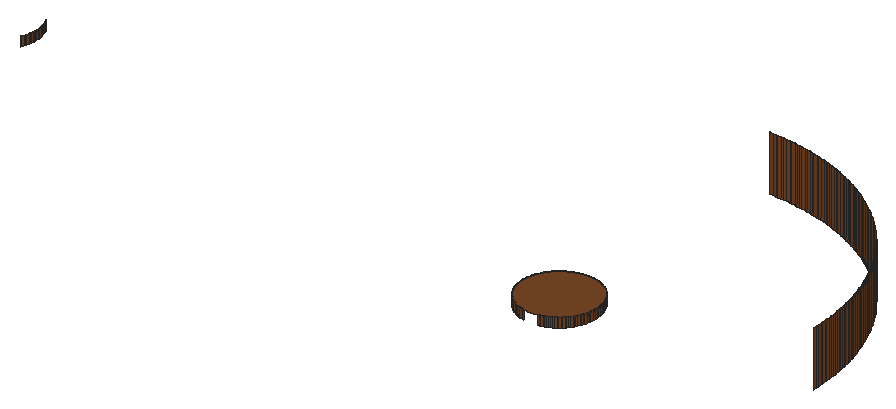
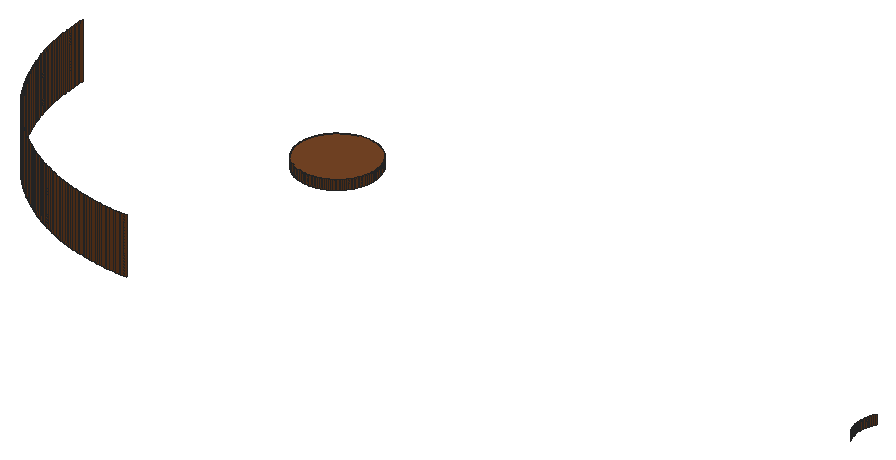
# SketchUp Ruby script. Lengths in inches.
U = 1.inch
M = Sketchup.active_model
def pt(a) = Geom::Point3d.new(a.map { |v| v * U })
def face(e, loops, mat)
  f = e.add_face(loops[0].map { |a| pt(a) })
  loops[1..].each { |l| e.add_face(l.map { |a| pt(a) }).erase! }
  f.material = f.back_material = mat if mat
  f
end
# faces: each face lists its corners as indices into pts; further lists are holes
def faces(e, pts, list, mat = nil) = list.each { |f| face(e, (f[0].is_a?(Array) ? f : [f]).map { |l| l.map { |i| pts[i] } }, mat) }
# xy, xz, yz: faces in a plane at the given z, y or x. An outline is a flat list of corners, or four numbers for a rectangle; further outlines are holes
def ring(l) = l.size == 4 ? [[l[0], l[1]], [l[2], l[1]], [l[2], l[3]], [l[0], l[3]]] : l.each_slice(2).to_a
def flat(e, list, mat, &to3) = list.each { |f| face(e, (f[0].is_a?(Array) ? f : [f]).map { |l| ring(l).map { |u, v| to3.(u, v) } }, mat) }
def xy(e, z, list, mat = nil) = flat(e, list, mat) { |x, y| [x, y, z] }
def xz(e, y, list, mat = nil) = flat(e, list, mat) { |x, z| [x, y, z] }
def yz(e, x, list, mat = nil) = flat(e, list, mat) { |y, z| [x, y, z] }
def lines(e, pts, list) = list.each { |a, b| e.add_line(pt(pts[a]), pt(pts[b])) }
# prism: a flat outline (further loops are holes) pulled along v
def prism(e, loops, v, mat = nil)
  f = face(e, loops, mat); d = Geom::Vector3d.new(v.map { |x| x * U })
  f.pushpull(f.normal.samedirection?(d) ? d.length : -d.length)
end
def box(e, o, s, mat = nil) = prism(e, [[o, [o[0] + s[0], o[1], o[2]], [o[0] + s[0], o[1] + s[1], o[2]], [o[0], o[1] + s[1], o[2]]]], [0, 0, s[2]], mat)
def at(x, y, z, deg = 0) = Geom::Transformation.translation(pt([x, y, z])) * Geom::Transformation.rotation(ORIGIN, Z_AXIS, deg.degrees)
def axes(o, x, y, z) = Geom::Transformation.new([*x, 0, *y, 0, *z, 0, *pt(o).to_a, 1])
def part(name) = M.definitions.add(name)
# library, detail: a bought-in or finely detailed component or shape, given as its bounding box
def library(name, o, s) = part(name).tap { |d| box(d.entities, o, s) }
def detail(e, o, s) = box(e.add_group.entities, o, s)
def put(e, d, t, mat = nil) = e.add_instance(d, t).tap { |i| i.material = mat if mat }
def group(e, t, mat = nil) = e.add_group.tap { |g| g.transformation = t; g.material = mat if mat }.entities
root = M.entities
M.materials.add("[Wood Veneer 01]3").color = [120, 70, 37]
xy(root,118.5,[[142.9,168,142.74,168.02,142.65,168.03,142.41,168.09,142.17,168.18,142.1,168.21,142.02,168.25,141.95,168.3,141.88,168.34,141.8125,168.39,141.75,168.44,141.68,168.5,141.62,168.55,141.5625,168.61,141.5,168.67,141.45,168.74,141.4,168.8,141.3,168.94,141.26,169.01,141.22,169.09,141.18,169.16,141.09,169.4,141.03,169.64,141.01,169.8,141,169.89,141,170.14,141.01,170.22,141.02,170.31,141.1,170.63,141.16,170.79,141.2,170.86,141.23,170.9375,141.27,171.01,141.47,171.29,141.52,171.35,141.64,171.47,141.7,171.52,141.77,171.58,141.84,171.625,141.9,171.67,141.98,171.72,142.05,171.76,142.125,171.8,142.2,171.83,142.44,171.92,142.6,171.96,142.68,171.97,142.76,171.99,142.85,171.99,142.93,172,143.1,172,143.26,171.98,143.35,171.97,143.59,171.91,143.83,171.82,143.9,171.79,143.98,171.75,144.05,171.7,144.12,171.66,144.1875,171.61,144.25,171.56,144.32,171.5,144.38,171.45,144.4375,171.39,144.5,171.33,144.55,171.26,144.6,171.2,144.7,171.06,144.74,170.99,144.78,170.91,144.82,170.84,144.91,170.6,144.97,170.36,144.99,170.2,145,170.11,145,169.86,144.99,169.78,144.98,169.69,144.9,169.37,144.84,169.21,144.8,169.14,144.77,169.0625,144.73,168.99,144.53,168.71,144.48,168.65,144.36,168.53,144.3,168.48,144.23,168.42,144.16,168.375,144.1,168.33,144.02,168.28,143.95,168.24,143.875,168.2,143.8,168.17,143.56,168.08,143.4,168.04,143.32,168.03,143.24,168.01,143.15,168.01,143.07,168]],"[Wood Veneer 01]3")
xz(root,171.99,[[142.76,118,142.85,118.5]],"[Wood Veneer 01]3")
xz(root,172,[[142.93,118,143.01,118.5],[143.01,118,143.1,118.5]],"[Wood Veneer 01]3")
xz(root,183,[[144,118,144.16,121],[144.16,118,144.3125,121]],"[Wood Veneer 01]3")
yz(root,111.5,[[173.86,118,173.94,118.5],[173.94,118,174.03,118.5],[174.03,118,174.11,118.5]],"[Wood Veneer 01]3")
yz(root,141,[[169.89,118,169.97,118.5],[169.97,118,170.06,118.5],[170.06,118,170.14,118.5]],"[Wood Veneer 01]3")
yz(root,145,[[169.86,118,169.94,118.5],[169.94,118,170.03,118.5],[170.03,118,170.11,118.5]],"[Wood Veneer 01]3")
yz(root,156,[[171,118,171.16,121],[171.16,118,171.3125,121]],"[Wood Veneer 01]3")
p = [[142.57,168.05,118],[142.49,168.07,118],[142.49,168.07,118.5],[142.57,168.05,118.5],[142.65,168.03,118],[142.65,168.03,118.5],
  [143.48,168.06,118],[143.4,168.04,118],[143.4,168.04,118.5],[143.48,168.06,118.5],[142.25,168.15,118],[142.17,168.18,118],
  [142.17,168.18,118.5],[142.25,168.15,118.5],[142.41,168.09,118],[142.33,168.12,118],[142.33,168.12,118.5],[142.41,168.09,118.5],
  [143.56,168.08,118],[143.56,168.08,118.5],[143.64,168.11,118],[143.64,168.11,118.5],[143.72,168.14,118],[143.72,168.14,118.5],
  [143.8,168.17,118],[143.8,168.17,118.5],[142.1,168.21,118],[142.02,168.25,118],[142.02,168.25,118.5],[142.1,168.21,118.5],
  [143.875,168.2,118],[143.875,168.2,118.5],[143.95,168.24,118],[143.95,168.24,118.5],[144.02,168.28,118],[144.02,168.28,118.5],
  [141.88,168.34,118],[141.8125,168.39,118],[141.8125,168.39,118.5],[141.88,168.34,118.5],[141.95,168.3,118],[141.95,168.3,118.5],
  [144.1,168.33,118],[144.1,168.33,118.5],[144.16,168.375,118],[144.16,168.375,118.5],[141.75,168.44,118],[141.75,168.44,118.5],
  [141.68,168.5,118],[141.68,168.5,118.5],[144.23,168.42,118],[144.23,168.42,118.5],[144.3,168.48,118],[144.3,168.48,118.5],
  [141.62,168.55,118],[141.62,168.55,118.5],[144.36,168.53,118],[144.36,168.53,118.5],[144.42,168.59,118],[144.42,168.59,118.5],
  [141.5625,168.61,118],[141.5,168.67,118],[141.5,168.67,118.5],[141.5625,168.61,118.5],[144.48,168.65,118],[144.48,168.65,118.5],
  [141.45,168.74,118],[141.4,168.8,118],[141.4,168.8,118.5],[141.45,168.74,118.5],[144.53,168.71,118],[144.53,168.71,118.5],
  [144.58,168.78,118],[144.58,168.78,118.5],[141.35,168.87,118],[141.35,168.87,118.5],[144.63,168.85,118],[144.63,168.85,118.5],
  [144.68,168.92,118],[144.68,168.92,118.5],[141.3,168.94,118],[141.3,168.94,118.5],[141.26,169.01,118],[141.26,169.01,118.5],
  [144.73,168.99,118],[144.73,168.99,118.5],[141.22,169.09,118],[141.22,169.09,118.5],[144.77,169.0625,118],[144.77,169.0625,118.5],
  [141.18,169.16,118],[141.18,169.16,118.5],[144.8,169.14,118],[144.8,169.14,118.5],[144.84,169.21,118],[144.84,169.21,118.5],
  [141.15,169.24,118],[141.12,169.32,118],[141.12,169.32,118.5],[141.15,169.24,118.5],[144.87,169.29,118],[144.87,169.29,118.5],
  [141.09,169.4,118],[141.09,169.4,118.5],[144.9,169.37,118],[144.9,169.37,118.5],[141.07,169.48,118],[141.07,169.48,118.5],
  [144.92,169.45,118],[144.92,169.45,118.5],[144.94,169.53,118],[144.94,169.53,118.5],[141.05,169.56,118],[141.05,169.56,118.5],
  [144.96,169.61,118],[144.96,169.61,118.5],[141.03,169.64,118],[141.03,169.64,118.5],[141.02,169.72,118],[141.02,169.72,118.5],
  [144.98,169.69,118],[144.98,169.69,118.5],[141.01,169.8,118],[141.01,169.8,118.5],[144.99,169.78,118],[144.99,169.78,118.5],
  [141,169.89,118],[141,169.89,118.5],[145,169.86,118],[145,169.86,118.5],[141,170.14,118],[141.01,170.22,118],
  [141.01,170.22,118.5],[141,170.14,118.5],[144.99,170.2,118],[145,170.11,118],[145,170.11,118.5],[144.99,170.2,118.5],
  [141.02,170.31,118],[141.02,170.31,118.5],[144.98,170.28,118],[144.98,170.28,118.5],[141.04,170.39,118],[141.04,170.39,118.5],
  [144.97,170.36,118],[144.97,170.36,118.5],[141.06,170.47,118],[141.06,170.47,118.5],[144.93,170.52,118],[144.95,170.44,118],
  [144.95,170.44,118.5],[144.93,170.52,118.5],[141.08,170.55,118],[141.08,170.55,118.5],[144.91,170.6,118],[144.91,170.6,118.5],
  [141.1,170.63,118],[141.1,170.63,118.5],[141.13,170.71,118],[141.13,170.71,118.5],[144.88,170.68,118],[144.88,170.68,118.5],
  [141.16,170.79,118],[141.16,170.79,118.5],[144.85,170.76,118],[144.85,170.76,118.5],[141.2,170.86,118],[141.2,170.86,118.5],
  [144.82,170.84,118],[144.82,170.84,118.5],[144.78,170.91,118],[144.78,170.91,118.5],[141.23,170.9375,118],[141.23,170.9375,118.5],
  [141.27,171.01,118],[141.27,171.01,118.5],[144.74,170.99,118],[144.74,170.99,118.5],[141.32,171.08,118],[141.32,171.08,118.5],
  [144.7,171.06,118],[144.7,171.06,118.5],[141.37,171.15,118],[141.37,171.15,118.5],[144.6,171.2,118],[144.65,171.13,118],
  [144.65,171.13,118.5],[144.6,171.2,118.5],[141.42,171.22,118],[141.42,171.22,118.5],[141.47,171.29,118],[141.47,171.29,118.5],
  [144.55,171.26,118],[144.55,171.26,118.5],[141.52,171.35,118],[141.52,171.35,118.5],[141.58,171.41,118],[141.58,171.41,118.5],
  [144.4375,171.39,118],[144.5,171.33,118],[144.5,171.33,118.5],[144.4375,171.39,118.5],[155.99,171.47,121],[156,171.3125,121],
  [156,171.3125,118],[155.99,171.47,118],[141.64,171.47,118],[141.64,171.47,118.5],[144.32,171.5,118],[144.38,171.45,118],
  [144.38,171.45,118.5],[144.32,171.5,118.5],[141.7,171.52,118],[141.7,171.52,118.5],[141.77,171.58,118],[141.77,171.58,118.5],
  [144.25,171.56,118],[144.25,171.56,118.5],[155.98,171.63,121],[155.98,171.63,118],[141.84,171.625,118],[141.84,171.625,118.5],
  [141.9,171.67,118],[141.9,171.67,118.5],[144.12,171.66,118],[144.1875,171.61,118],[144.1875,171.61,118.5],[144.12,171.66,118.5],
  [155.97,171.78,121],[155.97,171.78,118],[141.98,171.72,118],[141.98,171.72,118.5],[142.05,171.76,118],[142.05,171.76,118.5],
  [143.9,171.79,118],[143.98,171.75,118],[143.98,171.75,118.5],[143.9,171.79,118.5],[144.05,171.7,118],[144.05,171.7,118.5],
  [142.125,171.8,118],[142.125,171.8,118.5],[142.2,171.83,118],[142.2,171.83,118.5],[142.28,171.86,118],[142.28,171.86,118.5],
  [143.75,171.85,118],[143.83,171.82,118],[143.83,171.82,118.5],[143.75,171.85,118.5],[155.96,171.94,121],[155.96,171.94,118],
  [142.36,171.89,118],[142.36,171.89,118.5],[142.44,171.92,118],[142.44,171.92,118.5],[142.52,171.94,118],[142.52,171.94,118.5],
  [142.6,171.96,118],[142.6,171.96,118.5],[143.43,171.95,118],[143.51,171.93,118],[143.51,171.93,118.5],[143.43,171.95,118.5],
  [143.59,171.91,118],[143.59,171.91,118.5],[143.67,171.88,118],[143.67,171.88,118.5],[155.95,172.1,121],[155.95,172.1,118],
  [142.68,171.97,118],[142.68,171.97,118.5],[142.76,171.99,118],[142.76,171.99,118.5],[142.85,171.99,118],[142.93,172,118],
  [142.93,172,118.5],[142.85,171.99,118.5],[143.1,172,118],[143.18,171.99,118],[143.18,171.99,118.5],[143.1,172,118.5],
  [143.26,171.98,118],[143.26,171.98,118.5],[143.35,171.97,118],[143.35,171.97,118.5],[155.93,172.25,121],[155.93,172.25,118],
  [155.92,172.41,121],[155.92,172.41,118],[155.9,172.57,121],[155.9,172.57,118],[155.875,172.72,121],[155.875,172.72,118],
  [155.85,172.88,121],[155.85,172.88,118],[155.83,173.03,121],[155.83,173.03,118],[155.8,173.1875,121],[155.8,173.1875,118],
  [111.34,173.21,118],[111.3,173.14,118],[111.3,173.14,118.5],[111.34,173.21,118.5],[111.37,173.29,118],[111.37,173.29,118.5],
  [155.77,173.34,121],[155.77,173.34,118],[111.4,173.37,118],[111.4,173.37,118.5],[155.74,173.49,121],[155.74,173.49,118],
  [111.42,173.45,118],[111.42,173.45,118.5],[111.44,173.53,118],[111.44,173.53,118.5],[111.46,173.61,118],[111.46,173.61,118.5],
  [155.7,173.65,121],[155.7,173.65,118],[111.48,173.69,118],[111.48,173.69,118.5],[155.67,173.8,121],[155.67,173.8,118],
  [111.49,173.78,118],[111.49,173.78,118.5],[111.5,173.86,118],[111.5,173.86,118.5],[155.63,173.95,121],[155.63,173.95,118],
  [155.59,174.11,121],[155.59,174.11,118],[111.49,174.2,118],[111.5,174.11,118],[111.5,174.11,118.5],[111.49,174.2,118.5],
  [155.55,174.26,121],[155.55,174.26,118],[111.48,174.28,118],[111.48,174.28,118.5],[111.47,174.36,118],[111.47,174.36,118.5],
  [155.51,174.41,121],[155.51,174.41,118],[111.43,174.52,118],[111.45,174.44,118],[111.45,174.44,118.5],[111.43,174.52,118.5],
  [155.46,174.56,121],[155.46,174.56,118],[111.41,174.6,118],[111.41,174.6,118.5],[111.38,174.68,118],[111.38,174.68,118.5],
  [155.41,174.71,121],[155.41,174.71,118],[111.35,174.76,118],[111.35,174.76,118.5],[155.36,174.86,121],[155.36,174.86,118],
  [111.32,174.84,118],[111.32,174.84,118.5],[111.28,174.91,118],[111.28,174.91,118.5],[155.3125,175.01,121],[155.3125,175.01,118],
  [155.26,175.15,121],[155.26,175.15,118],[155.2,175.3,121],[155.2,175.3,118],[155.15,175.45,121],[155.15,175.45,118],
  [155.09,175.59,121],[155.09,175.59,118],[155.03,175.74,121],[155.03,175.74,118],[154.96,175.88,121],[154.96,175.88,118],
  [154.9,176.02,121],[154.9,176.02,118],[154.83,176.17,121],[154.83,176.17,118],[154.76,176.31,121],[154.76,176.31,118],
  [154.69,176.45,121],[154.69,176.45,118],[154.62,176.59,121],[154.62,176.59,118],[154.55,176.73,121],[154.55,176.73,118],
  [154.47,176.86,121],[154.47,176.86,118],[154.39,177,121],[154.39,177,118],[154.3125,177.14,121],[154.3125,177.14,118],
  [154.23,177.27,121],[154.23,177.27,118],[154.15,177.4,121],[154.15,177.4,118],[154.0625,177.54,121],[154.0625,177.54,118],
  [153.98,177.67,121],[153.98,177.67,118],[153.89,177.8,121],[153.89,177.8,118],[153.8,177.93,121],[153.8,177.93,118],
  [153.71,178.05,121],[153.71,178.05,118],[153.62,178.18,121],[153.62,178.18,118],[153.52,178.31,121],[153.52,178.31,118],
  [153.42,178.43,121],[153.42,178.43,118],[153.33,178.55,121],[153.33,178.55,118],[153.23,178.67,121],[153.23,178.67,118],
  [153.125,178.79,121],[153.125,178.79,118],[153.02,178.91,121],[153.02,178.91,118],[152.92,179.03,121],[152.92,179.03,118],
  [152.8125,179.15,121],[152.8125,179.15,118],[152.7,179.26,121],[152.7,179.26,118],[152.6,179.375,121],[152.6,179.375,118],
  [152.49,179.49,121],[152.49,179.49,118],[152.375,179.6,121],[152.375,179.6,118],[152.26,179.7,121],[152.26,179.7,118],
  [152.15,179.8125,121],[152.15,179.8125,118],[152.03,179.92,121],[152.03,179.92,118],[151.91,180.02,121],[151.91,180.02,118],
  [151.79,180.125,121],[151.79,180.125,118],[151.67,180.23,121],[151.67,180.23,118],[151.55,180.33,121],[151.55,180.33,118],
  [151.43,180.42,121],[151.43,180.42,118],[151.31,180.52,121],[151.31,180.52,118],[151.18,180.62,121],[151.18,180.62,118],
  [151.05,180.71,121],[151.05,180.71,118],[150.93,180.8,121],[150.93,180.8,118],[150.8,180.89,121],[150.8,180.89,118],
  [150.67,180.98,121],[150.67,180.98,118],[150.54,181.0625,121],[150.54,181.0625,118],[150.27,181.23,121],[150.4,181.15,121],
  [150.4,181.15,118],[150.27,181.23,118],[150.14,181.3125,121],[150.14,181.3125,118],[150,181.39,121],[150,181.39,118],
  [149.86,181.47,121],[149.86,181.47,118],[149.59,181.62,121],[149.73,181.55,121],[149.73,181.55,118],[149.59,181.62,118],
  [149.45,181.69,121],[149.45,181.69,118],[149.31,181.76,121],[149.31,181.76,118],[149.02,181.9,121],[149.17,181.83,121],
  [149.17,181.83,118],[149.02,181.9,118],[148.88,181.96,121],[148.88,181.96,118],[148.59,182.09,121],[148.74,182.03,121],
  [148.74,182.03,118],[148.59,182.09,118],[148.3,182.2,121],[148.45,182.15,121],[148.45,182.15,118],[148.3,182.2,118],
  [148.15,182.26,121],[148.15,182.26,118],[147.86,182.36,121],[148.01,182.3125,121],[148.01,182.3125,118],[147.86,182.36,118],
  [147.56,182.46,121],[147.71,182.41,121],[147.71,182.41,118],[147.56,182.46,118],[147.11,182.59,121],[147.26,182.55,121],
  [147.26,182.55,118],[147.11,182.59,118],[147.41,182.51,121],[147.41,182.51,118],[146.8,182.67,121],[146.95,182.63,121],
  [146.95,182.63,118],[146.8,182.67,118],[146.34,182.77,121],[146.49,182.74,121],[146.49,182.74,118],[146.34,182.77,118],
  [146.65,182.7,121],[146.65,182.7,118],[145.88,182.85,121],[146.03,182.83,121],[146.03,182.83,118],[145.88,182.85,118],
  [146.1875,182.8,121],[146.1875,182.8,118],[144.94,182.96,121],[145.1,182.95,121],[145.1,182.95,118],[144.94,182.96,118],
  [145.25,182.93,121],[145.25,182.93,118],[145.41,182.92,121],[145.41,182.92,118],[145.57,182.9,121],[145.57,182.9,118],
  [145.72,182.875,121],[145.72,182.875,118],[144.3125,183,121],[144.47,182.99,121],[144.47,182.99,118],[144.3125,183,118],
  [144.63,182.98,121],[144.63,182.98,118],[144.78,182.97,121],[144.78,182.97,118]]
faces(root,p,[[0,1,2,3],[4,0,3,5],[6,7,8,9],[10,11,12,13],[14,15,16,17],[15,10,13,16],[1,14,17,2],[18,6,9,19],
  [20,18,19,21],[22,20,21,23],[24,22,23,25],[26,27,28,29],[11,26,29,12],[30,24,25,31],[32,30,31,33],[34,32,33,35],
  [36,37,38,39],[40,36,39,41],[27,40,41,28],[42,34,35,43],[44,42,43,45],[37,46,47,38],[46,48,49,47],[50,44,45,51],
  [52,50,51,53],[48,54,55,49],[56,52,53,57],[58,56,57,59],[60,61,62,63],[54,60,63,55],[64,58,59,65],[66,67,68,69],
  [61,66,69,62],[70,64,65,71],[72,70,71,73],[67,74,75,68],[76,72,73,77],[78,76,77,79],[74,80,81,75],[80,82,83,81],
  [84,78,79,85],[82,86,87,83],[88,84,85,89],[86,90,91,87],[92,88,89,93],[94,92,93,95],[96,97,98,99],[90,96,99,91],
  [100,94,95,101],[97,102,103,98],[104,100,101,105],[102,106,107,103],[108,104,105,109],[110,108,109,111],[106,112,113,107],[114,110,111,115],
  [112,116,117,113],[116,118,119,117],[120,114,115,121],[118,122,123,119],[124,120,121,125],[122,126,127,123],[128,124,125,129],[130,131,132,133],
  [134,135,136,137],[131,138,139,132],[140,134,137,141],[138,142,143,139],[144,140,141,145],[142,146,147,143],[148,149,150,151],[149,144,145,150],
  [146,152,153,147],[154,148,151,155],[152,156,157,153],[156,158,159,157],[160,154,155,161],[158,162,163,159],[164,160,161,165],[162,166,167,163],
  [168,164,165,169],[170,168,169,171],[166,172,173,167],[172,174,175,173],[176,170,171,177],[174,178,179,175],[180,176,177,181],[178,182,183,179],
  [184,185,186,187],[185,180,181,186],[182,188,189,183],[188,190,191,189],[192,184,187,193],[190,194,195,191],[194,196,197,195],[198,199,200,201],
  [199,192,193,200],[202,203,204,205],[196,206,207,197],[208,209,210,211],[209,198,201,210],[206,212,213,207],[212,214,215,213],[216,208,211,217],
  [218,202,205,219],[214,220,221,215],[220,222,223,221],[224,225,226,227],[225,216,217,226],[228,218,219,229],[222,230,231,223],[230,232,233,231],
  [234,235,236,237],[238,224,227,239],[235,238,239,236],[232,240,241,233],[240,242,243,241],[242,244,245,243],[246,247,248,249],[247,234,237,248],
  [250,228,229,251],[244,252,253,245],[252,254,255,253],[254,256,257,255],[256,258,259,257],[260,261,262,263],[261,264,265,262],[264,266,267,265],
  [266,246,249,267],[268,250,251,269],[258,270,271,259],[270,272,273,271],[274,275,276,277],[278,279,280,281],[279,282,283,280],[284,260,263,285],
  [282,284,285,283],[286,268,269,287],[288,286,287,289],[290,288,289,291],[292,290,291,293],[294,292,293,295],[296,294,295,297],[298,296,297,299],
  [300,301,302,303],[304,300,303,305],[306,298,299,307],[308,304,305,309],[310,306,307,311],[312,308,309,313],[314,312,313,315],[316,314,315,317],
  [318,310,311,319],[320,316,317,321],[322,318,319,323],[324,320,321,325],[326,324,325,327],[328,322,323,329],[330,328,329,331],[332,333,334,335],
  [336,330,331,337],[338,332,335,339],[340,338,339,341],[342,336,337,343],[344,345,346,347],[345,340,341,346],[348,342,343,349],[350,344,347,351],
  [352,350,351,353],[354,348,349,355],[356,352,353,357],[358,354,355,359],[360,356,357,361],[362,360,361,363],[364,358,359,365],[366,364,365,367],
  [368,366,367,369],[370,368,369,371],[372,370,371,373],[374,372,373,375],[376,374,375,377],[378,376,377,379],[380,378,379,381],[382,380,381,383],
  [384,382,383,385],[386,384,385,387],[388,386,387,389],[390,388,389,391],[392,390,391,393],[394,392,393,395],[396,394,395,397],[398,396,397,399],
  [400,398,399,401],[402,400,401,403],[404,402,403,405],[406,404,405,407],[408,406,407,409],[410,408,409,411],[412,410,411,413],[414,412,413,415],
  [416,414,415,417],[418,416,417,419],[420,418,419,421],[422,420,421,423],[424,422,423,425],[426,424,425,427],[428,426,427,429],[430,428,429,431],
  [432,430,431,433],[434,432,433,435],[436,434,435,437],[438,436,437,439],[440,438,439,441],[442,440,441,443],[444,442,443,445],[446,444,445,447],
  [448,446,447,449],[450,448,449,451],[452,450,451,453],[454,452,453,455],[456,454,455,457],[458,456,457,459],[460,458,459,461],[462,460,461,463],
  [464,462,463,465],[466,467,468,469],[467,464,465,468],[470,466,469,471],[472,470,471,473],[474,472,473,475],[476,477,478,479],[477,474,475,478],
  [480,476,479,481],[482,480,481,483],[484,485,486,487],[485,482,483,486],[488,484,487,489],[490,491,492,493],[491,488,489,492],[494,495,496,497],
  [495,490,493,496],[498,494,497,499],[500,501,502,503],[501,498,499,502],[504,505,506,507],[505,500,503,506],[508,509,510,511],[509,512,513,510],
  [512,504,507,513],[514,515,516,517],[515,508,511,516],[518,519,520,521],[519,522,523,520],[522,514,517,523],[524,525,526,527],[525,528,529,526],
  [528,518,521,529],[530,531,532,533],[531,534,535,532],[534,536,537,535],[536,538,539,537],[538,540,541,539],[540,524,527,541],[542,543,544,545],
  [543,546,547,544],[546,548,549,547],[548,530,533,549]],"[Wood Veneer 01]3")
